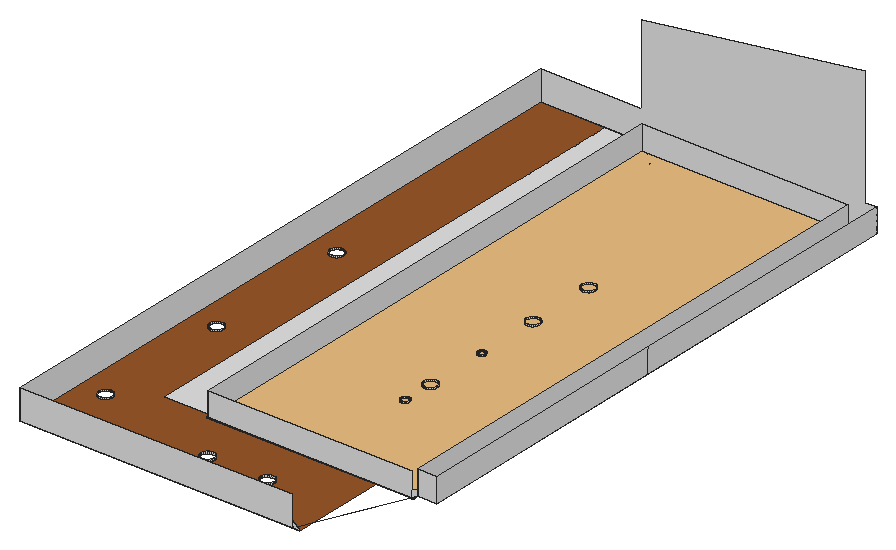
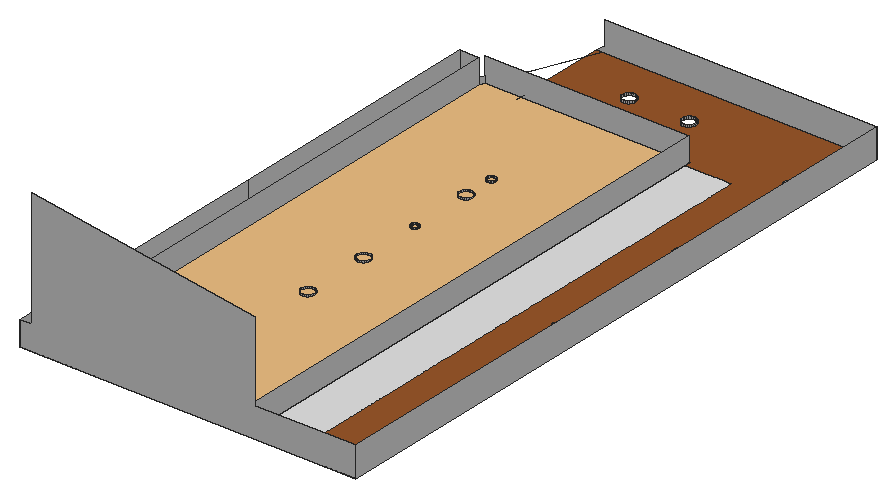
# SketchUp Ruby script. Lengths in inches.
U = 1.inch
M = Sketchup.active_model
def pt(a) = Geom::Point3d.new(a.map { |v| v * U })
def face(e, loops, mat)
  f = e.add_face(loops[0].map { |a| pt(a) })
  loops[1..].each { |l| e.add_face(l.map { |a| pt(a) }).erase! }
  f.material = f.back_material = mat if mat
  f
end
# faces: each face lists its corners as indices into pts; further lists are holes
def faces(e, pts, list, mat = nil) = list.each { |f| face(e, (f[0].is_a?(Array) ? f : [f]).map { |l| l.map { |i| pts[i] } }, mat) }
# xy, xz, yz: faces in a plane at the given z, y or x. An outline is a flat list of corners, or four numbers for a rectangle; further outlines are holes
def ring(l) = l.size == 4 ? [[l[0], l[1]], [l[2], l[1]], [l[2], l[3]], [l[0], l[3]]] : l.each_slice(2).to_a
def flat(e, list, mat, &to3) = list.each { |f| face(e, (f[0].is_a?(Array) ? f : [f]).map { |l| ring(l).map { |u, v| to3.(u, v) } }, mat) }
def xy(e, z, list, mat = nil) = flat(e, list, mat) { |x, y| [x, y, z] }
def xz(e, y, list, mat = nil) = flat(e, list, mat) { |x, z| [x, y, z] }
def yz(e, x, list, mat = nil) = flat(e, list, mat) { |y, z| [x, y, z] }
def lines(e, pts, list) = list.each { |a, b| e.add_line(pt(pts[a]), pt(pts[b])) }
# prism: a flat outline (further loops are holes) pulled along v
def prism(e, loops, v, mat = nil)
  f = face(e, loops, mat); d = Geom::Vector3d.new(v.map { |x| x * U })
  f.pushpull(f.normal.samedirection?(d) ? d.length : -d.length)
end
def box(e, o, s, mat = nil) = prism(e, [[o, [o[0] + s[0], o[1], o[2]], [o[0] + s[0], o[1] + s[1], o[2]], [o[0], o[1] + s[1], o[2]]]], [0, 0, s[2]], mat)
def at(x, y, z, deg = 0) = Geom::Transformation.translation(pt([x, y, z])) * Geom::Transformation.rotation(ORIGIN, Z_AXIS, deg.degrees)
def axes(o, x, y, z) = Geom::Transformation.new([*x, 0, *y, 0, *z, 0, *pt(o).to_a, 1])
def part(name) = M.definitions.add(name)
# library, detail: a bought-in or finely detailed component or shape, given as its bounding box
def library(name, o, s) = part(name).tap { |d| box(d.entities, o, s) }
def detail(e, o, s) = box(e.add_group.entities, o, s)
def put(e, d, t, mat = nil) = e.add_instance(d, t).tap { |i| i.material = mat if mat }
def group(e, t, mat = nil) = e.add_group.tap { |g| g.transformation = t; g.material = mat if mat }.entities
root = M.entities
M.materials.add("[Color M03]").color = [226, 226, 226]
M.materials.add("[Wood Cherry Original]2").color = [152, 86, 42]
c1 = library("Mesh Light\#9",[-0.5,-0.5,-0.1],[1,1,0.2])
xy(root,306.98,[[533.7,242.01,540.52,242.01,540.52,710.07,355.97,710.07,355.97,709.81,533.7,709.81]])
xy(root,306.98,[[500.59,227.88,500.59,232.04,533.7,232.04,531.81,227.88],[309.43,232.04,350.6,232.04,350.6,709.81,355.97,709.81,355.97,710.07,540.52,710.07,540.52,242.01,533.7,242.01,533.7,232.04,550.5,232.04,550.5,720.04,309.43,720.04],[350.6,232.04,363.68,232.04,363.68,242.01,355.97,242.01,355.97,709.81,350.6,709.81],[489.29,232.04,533.7,242.01],[[374.01,238.2,374.01,252.33,366.29,252.33,366.29,699.48,523.375,699.48,523.375,252.33,478.97,252.33,478.97,238.2],[442.84,467.81,444.39,468.02,445.84,468.62,447.08,469.57,448.03,470.81,448.63,472.26,448.84,473.81,448.63,475.37,448.03,476.81,447.08,478.06,445.84,479.01,444.39,479.61,442.84,479.81,441.28,479.61,439.84,479.01,438.59,478.06,437.64,476.81,437.04,475.37,436.84,473.81,437.04,472.26,437.64,470.81,438.59,469.57,439.84,468.62,441.28,468.02],[442.84,354.11,444.39,354.3125,445.84,354.91,447.08,355.87,448.03,357.11,448.63,358.56,448.84,360.11,448.63,361.66,448.03,363.11,447.08,364.35,445.84,365.31,444.39,365.9,442.84,366.11,441.28,365.9,439.84,365.31,438.59,364.35,437.64,363.11,437.04,361.66,436.84,360.11,437.04,358.56,437.64,357.11,438.59,355.87,439.84,354.91,441.28,354.3125],[442.84,529.49,444.39,529.7,445.84,530.3,447.08,531.25,448.03,532.49,448.63,533.94,448.84,535.49,448.63,537.05,448.03,538.49,447.08,539.74,445.84,540.69,444.39,541.29,442.84,541.49,441.28,541.29,439.84,540.69,438.59,539.74,437.64,538.49,437.04,537.05,436.84,535.49,437.04,533.94,437.64,532.49,438.59,531.25,439.84,530.3,441.28,529.7],[442.84,328.26,443.82,328.39,444.74,328.77,445.52,329.37,446.13,330.16,446.51,331.07,446.64,332.06,446.51,333.04,446.13,333.96,445.52,334.74,444.74,335.35,443.82,335.73,442.84,335.86,441.85,335.73,440.9375,335.35,440.15,334.74,439.54,333.96,439.17,333.04,439.04,332.06,439.17,331.07,439.54,330.16,440.15,329.37,440.9375,328.77,441.85,328.39],[442.84,413.34,443.73,413.46,444.55,413.8,445.27,414.35,445.8125,415.0625,446.16,415.89,446.27,416.78,446.16,417.67,445.8125,418.5,445.27,419.21,444.55,419.76,443.73,420.1,442.84,420.22,441.95,420.1,441.12,419.76,440.41,419.21,439.86,418.5,439.52,417.67,439.4,416.78,439.52,415.89,439.86,415.0625,440.41,414.35,441.12,413.8,441.95,413.46]]],"[Color M03]")
xy(root,306.98,[[[252.37,143.16,252.37,720.04,309.43,720.04,309.43,232.04,350.6,232.04,350.6,227.88,500.59,227.88,500.59,143.16],[275.74,459.14,277.29,459.35,278.74,459.95,279.98,460.9,280.9375,462.14,281.54,463.59,281.74,465.14,281.54,466.7,280.9375,468.14,279.98,469.39,278.74,470.34,277.29,470.94,275.74,471.14,274.1875,470.94,272.74,470.34,271.5,469.39,270.55,468.14,269.95,466.7,269.74,465.14,269.95,463.59,270.55,462.14,271.5,460.9,272.74,459.95,274.1875,459.35],[275.74,325.61,277.29,325.8125,278.74,326.41,279.98,327.37,280.9375,328.61,281.54,330.06,281.74,331.61,281.54,333.16,280.9375,334.61,279.98,335.85,278.74,336.8,277.29,337.4,275.74,337.61,274.1875,337.4,272.74,336.8,271.5,335.85,270.55,334.61,269.95,333.16,269.74,331.61,269.95,330.06,270.55,328.61,271.5,327.37,272.74,326.41,274.1875,325.8125],[439.47,177.38,441.02,177.59,442.47,178.1875,443.71,179.14,444.67,180.38,445.26,181.83,445.47,183.38,445.26,184.9375,444.67,186.38,443.71,187.625,442.47,188.58,441.02,189.18,439.47,189.38,437.92,189.18,436.47,188.58,435.23,187.625,434.27,186.38,433.67,184.9375,433.47,183.38,433.67,181.83,434.27,180.38,435.23,179.14,436.47,178.1875,437.92,177.59],[276.26,202.57,277.79,202.91,279.18,203.63,280.33,204.6875,281.18,206.01,281.65,207.5,281.72,209.07,281.38,210.6,280.66,211.99,279.6,213.14,278.28,213.98,276.79,214.46,275.22,214.53,273.69,214.1875,272.3,213.47,271.15,212.41,270.31,211.09,269.83,209.6,269.76,208.03,270.1,206.5,270.82,205.11,271.88,203.96,273.2,203.11,274.69,202.64],[386.3125,177.38,387.87,177.59,389.3125,178.1875,390.56,179.14,391.51,180.38,392.11,181.83,392.3125,183.38,392.11,184.9375,391.51,186.38,390.56,187.625,389.3125,188.58,387.87,189.18,386.3125,189.38,384.76,189.18,383.3125,188.58,382.07,187.625,381.12,186.38,380.52,184.9375,380.3125,183.38,380.52,181.83,381.12,180.38,382.07,179.14,383.3125,178.1875,384.76,177.59]]],"[Wood Cherry Original]2")
xz(root,143.16,[[252.37,306.98,500.59,306.98,493.34,312.98,493.34,333.29,252.37,333.29]],"[Color M03]")
xz(root,227.88,[[350.6,306.98,531.81,328.48]],"[Color M03]")
xz(root,232.04,[[533.7,306.98,550.5,328.48]],"[Color M03]")
xz(root,709.81,[[350.6,306.98,533.7,328.48]],"[Color M03]")
xz(root,720.04,[[252.37,306.98,252.37,333.29,342.34,333.29,342.34,403.74,540.65,432.98,540.65,328.48,550.5,328.48,550.5,306.98]],"[Color M03]")
yz(root,252.37,[[143.16,306.98,720.04,333.29]],"[Color M03]")
yz(root,350.6,[[227.88,306.98,709.81,328.48]],"[Color M03]")
yz(root,533.7,[[232.04,306.98,709.81,328.48]],"[Color M03]")
yz(root,550.5,[[232.04,306.98,466.93,328.48],[466.93,306.98,720.04,328.48]],"[Color M03]")
p = [[386.3125,177.38,306.98],[384.76,177.59,306.98],[384.76,177.59,308.86],[386.3125,177.38,308.86],[387.87,177.59,306.98],[387.87,177.59,308.86],
  [439.47,177.38,306.98],[437.92,177.59,306.98],[437.92,177.59,308.86],[439.47,177.38,308.86],[441.02,177.59,306.98],[441.02,177.59,308.86],
  [383.3125,178.1875,306.98],[383.3125,178.1875,308.86],[389.3125,178.1875,306.98],[389.3125,178.1875,308.86],[436.47,178.1875,306.98],[436.47,178.1875,308.86],
  [442.47,178.1875,306.98],[442.47,178.1875,308.86],[382.07,179.14,306.98],[382.07,179.14,308.86],[390.56,179.14,306.98],[390.56,179.14,308.86],
  [435.23,179.14,306.98],[435.23,179.14,308.86],[443.71,179.14,306.98],[443.71,179.14,308.86],[381.12,180.38,306.98],[381.12,180.38,308.86],
  [391.51,180.38,306.98],[391.51,180.38,308.86],[434.27,180.38,306.98],[434.27,180.38,308.86],[444.67,180.38,306.98],[444.67,180.38,308.86],
  [380.52,181.83,306.98],[380.52,181.83,308.86],[392.11,181.83,306.98],[392.11,181.83,308.86],[433.67,181.83,306.98],[433.67,181.83,308.86],
  [445.26,181.83,306.98],[445.26,181.83,308.86],[380.3125,183.38,306.98],[380.3125,183.38,308.86],[392.3125,183.38,306.98],[392.3125,183.38,308.86],
  [433.47,183.38,306.98],[433.47,183.38,308.86],[445.47,183.38,306.98],[445.47,183.38,308.86],[380.52,184.9375,306.98],[380.52,184.9375,308.86],
  [392.11,184.9375,306.98],[392.11,184.9375,308.86],[433.67,184.9375,306.98],[433.67,184.9375,308.86],[445.26,184.9375,306.98],[445.26,184.9375,308.86],
  [381.12,186.38,306.98],[381.12,186.38,308.86],[391.51,186.38,306.98],[391.51,186.38,308.86],[434.27,186.38,306.98],[434.27,186.38,308.86],
  [444.67,186.38,306.98],[444.67,186.38,308.86],[382.07,187.625,306.98],[382.07,187.625,308.86],[390.56,187.625,306.98],[390.56,187.625,308.86],
  [435.23,187.625,306.98],[435.23,187.625,308.86],[443.71,187.625,306.98],[443.71,187.625,308.86],[383.3125,188.58,306.98],[383.3125,188.58,308.86],
  [389.3125,188.58,306.98],[389.3125,188.58,308.86],[436.47,188.58,306.98],[436.47,188.58,308.86],[442.47,188.58,306.98],[442.47,188.58,308.86],
  [384.76,189.18,306.98],[384.76,189.18,308.86],[387.87,189.18,306.98],[387.87,189.18,308.86],[437.92,189.18,306.98],[437.92,189.18,308.86],
  [441.02,189.18,306.98],[441.02,189.18,308.86],[386.3125,189.38,306.98],[386.3125,189.38,308.86],[439.47,189.38,306.98],[439.47,189.38,308.86],
  [274.69,202.64,306.98],[273.2,203.11,306.98],[273.2,203.11,308.04],[274.69,202.64,308.04],[276.26,202.57,306.98],[276.26,202.57,308.04],
  [277.79,202.91,306.98],[277.79,202.91,308.04],[279.18,203.63,306.98],[279.18,203.63,308.04],[271.88,203.96,306.98],[271.88,203.96,308.04],
  [280.33,204.6875,306.98],[280.33,204.6875,308.04],[270.82,205.11,306.98],[270.82,205.11,308.04],[281.18,206.01,306.98],[281.18,206.01,308.04],
  [270.1,206.5,306.98],[270.1,206.5,308.04],[281.65,207.5,306.98],[281.65,207.5,308.04],[269.76,208.03,306.98],[269.76,208.03,308.04],
  [281.72,209.07,306.98],[281.72,209.07,308.04],[269.83,209.6,306.98],[269.83,209.6,308.04],[281.38,210.6,306.98],[281.38,210.6,308.04],
  [270.31,211.09,306.98],[270.31,211.09,308.04],[280.66,211.99,306.98],[280.66,211.99,308.04],[271.15,212.41,306.98],[271.15,212.41,308.04],
  [279.6,213.14,306.98],[279.6,213.14,308.04],[272.3,213.47,306.98],[272.3,213.47,308.04],[278.28,213.98,306.98],[278.28,213.98,308.04],
  [273.69,214.1875,306.98],[273.69,214.1875,308.04],[276.79,214.46,306.98],[276.79,214.46,308.04],[275.22,214.53,306.98],[275.22,214.53,308.04],
  [533.7,232.04,306.98],[533.7,232.04,312.98],[531.81,227.88,312.98],[531.81,227.88,306.98],[275.74,325.61,306.98],[274.1875,325.8125,306.98],
  [274.1875,325.8125,308.04],[275.74,325.61,308.04],[277.29,325.8125,306.98],[277.29,325.8125,308.04],[272.74,326.41,306.98],[272.74,326.41,308.04],
  [278.74,326.41,306.98],[278.74,326.41,308.04],[271.5,327.37,306.98],[271.5,327.37,308.04],[279.98,327.37,306.98],[279.98,327.37,308.04],
  [270.55,328.61,306.98],[270.55,328.61,308.04],[280.9375,328.61,306.98],[280.9375,328.61,308.04],[442.84,328.26,306.98],[441.85,328.39,306.98],
  [441.85,328.39,308.17],[442.84,328.26,308.17],[443.82,328.39,306.98],[443.82,328.39,308.17],[440.9375,328.77,306.98],[440.9375,328.77,308.17],
  [444.74,328.77,306.98],[444.74,328.77,308.17],[269.95,330.06,306.98],[269.95,330.06,308.04],[281.54,330.06,306.98],[281.54,330.06,308.04],
  [440.15,329.37,306.98],[440.15,329.37,308.17],[445.52,329.37,306.98],[445.52,329.37,308.17],[439.54,330.16,306.98],[439.54,330.16,308.17],
  [446.13,330.16,306.98],[446.13,330.16,308.17],[269.74,331.61,306.98],[269.74,331.61,308.04],[281.74,331.61,306.98],[281.74,331.61,308.04],
  [439.17,331.07,306.98],[439.17,331.07,308.17],[446.51,331.07,306.98],[446.51,331.07,308.17],[439.04,332.06,306.98],[439.04,332.06,308.17],
  [446.64,332.06,306.98],[446.64,332.06,308.17],[269.95,333.16,306.98],[269.95,333.16,308.04],[281.54,333.16,306.98],[281.54,333.16,308.04],
  [439.17,333.04,306.98],[439.17,333.04,308.17],[446.51,333.04,306.98],[446.51,333.04,308.17],[439.54,333.96,306.98],[439.54,333.96,308.17],
  [446.13,333.96,306.98],[446.13,333.96,308.17],[270.55,334.61,306.98],[270.55,334.61,308.04],[280.9375,334.61,306.98],[280.9375,334.61,308.04],
  [440.15,334.74,306.98],[440.15,334.74,308.17],[445.52,334.74,306.98],[445.52,334.74,308.17],[271.5,335.85,306.98],[271.5,335.85,308.04],
  [279.98,335.85,306.98],[279.98,335.85,308.04],[440.9375,335.35,306.98],[440.9375,335.35,308.17],[444.74,335.35,306.98],[444.74,335.35,308.17],
  [441.85,335.73,306.98],[441.85,335.73,308.17],[443.82,335.73,306.98],[443.82,335.73,308.17],[442.84,335.86,306.98],[442.84,335.86,308.17],
  [272.74,336.8,306.98],[272.74,336.8,308.04],[278.74,336.8,306.98],[278.74,336.8,308.04],[274.1875,337.4,306.98],[274.1875,337.4,308.04],
  [277.29,337.4,306.98],[277.29,337.4,308.04],[275.74,337.61,306.98],[275.74,337.61,308.04],[442.84,354.11,306.98],[441.28,354.3125,306.98],
  [441.28,354.3125,308.17],[442.84,354.11,308.17],[444.39,354.3125,306.98],[444.39,354.3125,308.17],[439.84,354.91,306.98],[439.84,354.91,308.17],
  [445.84,354.91,306.98],[445.84,354.91,308.17],[438.59,355.87,306.98],[438.59,355.87,308.17],[447.08,355.87,306.98],[447.08,355.87,308.17],
  [437.64,357.11,306.98],[437.64,357.11,308.17],[448.03,357.11,306.98],[448.03,357.11,308.17],[437.04,358.56,306.98],[437.04,358.56,308.17],
  [448.63,358.56,306.98],[448.63,358.56,308.17],[436.84,360.11,306.98],[436.84,360.11,308.17],[448.84,360.11,306.98],[448.84,360.11,308.17],
  [437.04,361.66,306.98],[437.04,361.66,308.17],[448.63,361.66,306.98],[448.63,361.66,308.17],[437.64,363.11,306.98],[437.64,363.11,308.17],
  [448.03,363.11,306.98],[448.03,363.11,308.17],[438.59,364.35,306.98],[438.59,364.35,308.17],[447.08,364.35,306.98],[447.08,364.35,308.17],
  [439.84,365.31,306.98],[439.84,365.31,308.17],[445.84,365.31,306.98],[445.84,365.31,308.17],[441.28,365.9,306.98],[441.28,365.9,308.17],
  [444.39,365.9,306.98],[444.39,365.9,308.17],[442.84,366.11,306.98],[442.84,366.11,308.17],[442.84,413.34,306.98],[441.95,413.46,306.98],
  [441.95,413.46,308.17],[442.84,413.34,308.17],[443.73,413.46,306.98],[443.73,413.46,308.17],[441.12,413.8,306.98],[441.12,413.8,308.17],
  [444.55,413.8,306.98],[444.55,413.8,308.17],[440.41,414.35,306.98],[440.41,414.35,308.17],[445.27,414.35,306.98],[445.27,414.35,308.17],
  [439.86,415.0625,306.98],[439.86,415.0625,308.17],[445.8125,415.0625,306.98],[445.8125,415.0625,308.17],[439.52,415.89,306.98],[439.52,415.89,308.17],
  [446.16,415.89,306.98],[446.16,415.89,308.17],[439.4,416.78,306.98],[439.4,416.78,308.17],[446.27,416.78,306.98],[446.27,416.78,308.17],
  [439.52,417.67,306.98],[439.52,417.67,308.17],[446.16,417.67,306.98],[446.16,417.67,308.17],[439.86,418.5,306.98],[439.86,418.5,308.17],
  [445.8125,418.5,306.98],[445.8125,418.5,308.17],[440.41,419.21,306.98],[440.41,419.21,308.17],[445.27,419.21,306.98],[445.27,419.21,308.17],
  [441.12,419.76,306.98],[441.12,419.76,308.17],[444.55,419.76,306.98],[444.55,419.76,308.17],[441.95,420.1,306.98],[441.95,420.1,308.17],
  [443.73,420.1,306.98],[443.73,420.1,308.17],[442.84,420.22,306.98],[442.84,420.22,308.17],[275.74,459.14,306.98],[274.1875,459.35,306.98],
  [274.1875,459.35,308.04],[275.74,459.14,308.04],[277.29,459.35,306.98],[277.29,459.35,308.04],[272.74,459.95,306.98],[272.74,459.95,308.04],
  [278.74,459.95,306.98],[278.74,459.95,308.04],[271.5,460.9,306.98],[271.5,460.9,308.04],[279.98,460.9,306.98],[279.98,460.9,308.04],
  [270.55,462.14,306.98],[270.55,462.14,308.04],[280.9375,462.14,306.98],[280.9375,462.14,308.04],[269.95,463.59,306.98],[269.95,463.59,308.04],
  [281.54,463.59,306.98],[281.54,463.59,308.04],[269.74,465.14,306.98],[269.74,465.14,308.04],[281.74,465.14,306.98],[281.74,465.14,308.04],
  [269.95,466.7,306.98],[269.95,466.7,308.04],[281.54,466.7,306.98],[281.54,466.7,308.04],[270.55,468.14,306.98],[270.55,468.14,308.04],
  [280.9375,468.14,306.98],[280.9375,468.14,308.04],[442.84,467.81,306.98],[441.28,468.02,306.98],[441.28,468.02,308.17],[442.84,467.81,308.17],
  [444.39,468.02,306.98],[444.39,468.02,308.17],[439.84,468.62,306.98],[439.84,468.62,308.17],[445.84,468.62,306.98],[445.84,468.62,308.17],
  [271.5,469.39,306.98],[271.5,469.39,308.04],[279.98,469.39,306.98],[279.98,469.39,308.04],[438.59,469.57,306.98],[438.59,469.57,308.17],
  [447.08,469.57,306.98],[447.08,469.57,308.17],[272.74,470.34,306.98],[272.74,470.34,308.04],[278.74,470.34,306.98],[278.74,470.34,308.04],
  [437.64,470.81,306.98],[437.64,470.81,308.17],[448.03,470.81,306.98],[448.03,470.81,308.17],[274.1875,470.94,306.98],[274.1875,470.94,308.04],
  [277.29,470.94,306.98],[277.29,470.94,308.04],[437.04,472.26,306.98],[437.04,472.26,308.17],[448.63,472.26,306.98],[448.63,472.26,308.17],
  [275.74,471.14,306.98],[275.74,471.14,308.04],[436.84,473.81,306.98],[436.84,473.81,308.17],[448.84,473.81,306.98],[448.84,473.81,308.17],
  [437.04,475.37,306.98],[437.04,475.37,308.17],[448.63,475.37,306.98],[448.63,475.37,308.17],[437.64,476.81,306.98],[437.64,476.81,308.17],
  [448.03,476.81,306.98],[448.03,476.81,308.17],[438.59,478.06,306.98],[438.59,478.06,308.17],[447.08,478.06,306.98],[447.08,478.06,308.17],
  [439.84,479.01,306.98],[439.84,479.01,308.17],[445.84,479.01,306.98],[445.84,479.01,308.17],[441.28,479.61,306.98],[441.28,479.61,308.17],
  [444.39,479.61,306.98],[444.39,479.61,308.17],[442.84,479.81,306.98],[442.84,479.81,308.17],[442.84,529.49,306.98],[441.28,529.7,306.98],
  [441.28,529.7,308.17],[442.84,529.49,308.17],[444.39,529.7,306.98],[444.39,529.7,308.17],[439.84,530.3,306.98],[439.84,530.3,308.17],
  [445.84,530.3,306.98],[445.84,530.3,308.17],[438.59,531.25,306.98],[438.59,531.25,308.17],[447.08,531.25,306.98],[447.08,531.25,308.17],
  [437.64,532.49,306.98],[437.64,532.49,308.17],[448.03,532.49,306.98],[448.03,532.49,308.17],[437.04,533.94,306.98],[437.04,533.94,308.17],
  [448.63,533.94,306.98],[448.63,533.94,308.17],[436.84,535.49,306.98],[436.84,535.49,308.17],[448.84,535.49,306.98],[448.84,535.49,308.17],
  [437.04,537.05,306.98],[437.04,537.05,308.17],[448.63,537.05,306.98],[448.63,537.05,308.17],[437.64,538.49,306.98],[437.64,538.49,308.17],
  [448.03,538.49,306.98],[448.03,538.49,308.17],[438.59,539.74,306.98],[438.59,539.74,308.17],[447.08,539.74,306.98],[447.08,539.74,308.17],
  [439.84,540.69,306.98],[439.84,540.69,308.17],[445.84,540.69,306.98],[445.84,540.69,308.17],[441.28,541.29,306.98],[441.28,541.29,308.17],
  [444.39,541.29,306.98],[444.39,541.29,308.17],[442.84,541.49,306.98],[442.84,541.49,308.17],[493.34,232.04,312.98],[500.59,232.04,306.98],
  [494.94,142.51,307.44],[493.34,143.16,312.98]]
faces(root,p,[[0,1,2,3],[4,0,3,5],[6,7,8,9],[10,6,9,11],[1,12,13,2],[14,4,5,15],[7,16,17,8],[18,10,11,19],
  [12,20,21,13],[22,14,15,23],[16,24,25,17],[26,18,19,27],[20,28,29,21],[30,22,23,31],[24,32,33,25],[34,26,27,35],
  [28,36,37,29],[38,30,31,39],[32,40,41,33],[42,34,35,43],[36,44,45,37],[46,38,39,47],[40,48,49,41],[50,42,43,51],
  [44,52,53,45],[54,46,47,55],[48,56,57,49],[58,50,51,59],[52,60,61,53],[62,54,55,63],[56,64,65,57],[66,58,59,67],
  [60,68,69,61],[70,62,63,71],[64,72,73,65],[74,66,67,75],[68,76,77,69],[78,70,71,79],[72,80,81,73],[82,74,75,83],
  [76,84,85,77],[86,78,79,87],[80,88,89,81],[90,82,83,91],[84,92,93,85],[92,86,87,93],[88,94,95,89],[94,90,91,95],
  [96,97,98,99],[100,96,99,101],[102,100,101,103],[104,102,103,105],[97,106,107,98],[108,104,105,109],[106,110,111,107],[112,108,109,113],
  [110,114,115,111],[116,112,113,117],[114,118,119,115],[120,116,117,121],[118,122,123,119],[124,120,121,125],[122,126,127,123],[128,124,125,129],
  [126,130,131,127],[132,128,129,133],[130,134,135,131],[136,132,133,137],[134,138,139,135],[140,136,137,141],[138,142,143,139],[142,140,141,143],
  [144,145,146,147],[148,149,150,151],[152,148,151,153],[149,154,155,150],[156,152,153,157],[154,158,159,155],[160,156,157,161],[158,162,163,159],
  [164,160,161,165],[166,167,168,169],[170,166,169,171],[167,172,173,168],[174,170,171,175],[162,176,177,163],[178,164,165,179],[172,180,181,173],
  [182,174,175,183],[180,184,185,181],[186,182,183,187],[176,188,189,177],[190,178,179,191],[184,192,193,185],[194,186,187,195],[192,196,197,193],
  [198,194,195,199],[188,200,201,189],[202,190,191,203],[196,204,205,197],[206,198,199,207],[204,208,209,205],[210,206,207,211],[200,212,213,201],
  [214,202,203,215],[208,216,217,209],[218,210,211,219],[212,220,221,213],[222,214,215,223],[216,224,225,217],[226,218,219,227],[224,228,229,225],
  [230,226,227,231],[228,232,233,229],[232,230,231,233],[220,234,235,221],[236,222,223,237],[234,238,239,235],[240,236,237,241],[238,242,243,239],
  [242,240,241,243],[244,245,246,247],[248,244,247,249],[245,250,251,246],[252,248,249,253],[250,254,255,251],[256,252,253,257],[254,258,259,255],
  [260,256,257,261],[258,262,263,259],[264,260,261,265],[262,266,267,263],[268,264,265,269],[266,270,271,267],[272,268,269,273],[270,274,275,271],
  [276,272,273,277],[274,278,279,275],[280,276,277,281],[278,282,283,279],[284,280,281,285],[282,286,287,283],[288,284,285,289],[286,290,291,287],
  [290,288,289,291],[292,293,294,295],[296,292,295,297],[293,298,299,294],[300,296,297,301],[298,302,303,299],[304,300,301,305],[302,306,307,303],
  [308,304,305,309],[306,310,311,307],[312,308,309,313],[310,314,315,311],[316,312,313,317],[314,318,319,315],[320,316,317,321],[318,322,323,319],
  [324,320,321,325],[322,326,327,323],[328,324,325,329],[326,330,331,327],[332,328,329,333],[330,334,335,331],[336,332,333,337],[334,338,339,335],
  [338,336,337,339],[340,341,342,343],[344,340,343,345],[341,346,347,342],[348,344,345,349],[346,350,351,347],[352,348,349,353],[350,354,355,351],
  [356,352,353,357],[354,358,359,355],[360,356,357,361],[358,362,363,359],[364,360,361,365],[362,366,367,363],[368,364,365,369],[366,370,371,367],
  [372,368,369,373],[374,375,376,377],[378,374,377,379],[375,380,381,376],[382,378,379,383],[370,384,385,371],[386,372,373,387],[380,388,389,381],
  [390,382,383,391],[384,392,393,385],[394,386,387,395],[388,396,397,389],[398,390,391,399],[392,400,401,393],[402,394,395,403],[396,404,405,397],
  [406,398,399,407],[400,408,409,401],[408,402,403,409],[404,410,411,405],[412,406,407,413],[410,414,415,411],[416,412,413,417],[414,418,419,415],
  [420,416,417,421],[418,422,423,419],[424,420,421,425],[422,426,427,423],[428,424,425,429],[426,430,431,427],[432,428,429,433],[430,434,435,431],
  [434,432,433,435],[436,437,438,439],[440,436,439,441],[437,442,443,438],[444,440,441,445],[442,446,447,443],[448,444,445,449],[446,450,451,447],
  [452,448,449,453],[450,454,455,451],[456,452,453,457],[454,458,459,455],[460,456,457,461],[458,462,463,459],[464,460,461,465],[462,466,467,463],
  [468,464,465,469],[466,470,471,467],[472,468,469,473],[470,474,475,471],[476,472,473,477],[474,478,479,475],[480,476,477,481],[478,482,483,479],
  [482,480,481,483]],"[Color M03]")
lines(root,p,[[484,485],[144,486],[486,487]])
g1 = group(root,at(350.6,227.88,306.98))
xy(g1,0,[[[0,0,0,4.16,13.09,4.16,13.09,14.13,5.375,14.13,5.375,481.93,183.1,481.93,183.1,14.13,138.69,14.13,138.69,4.16,149.99,4.16,149.99,0],[23.41,10.32,128.37,10.32,128.37,24.46,172.78,24.46,172.78,471.61,15.7,471.61,15.7,24.46,23.41,24.46]]],"[Color M03]")
put(g1,c1,axes([91.55,240.96,0],[184.10215,0,0],[0,482.92851,0],[0,0,1]))
